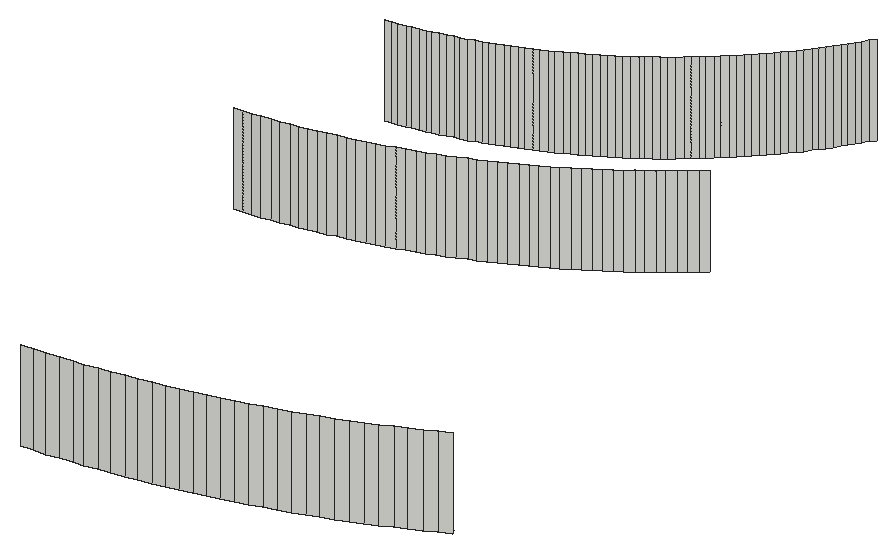
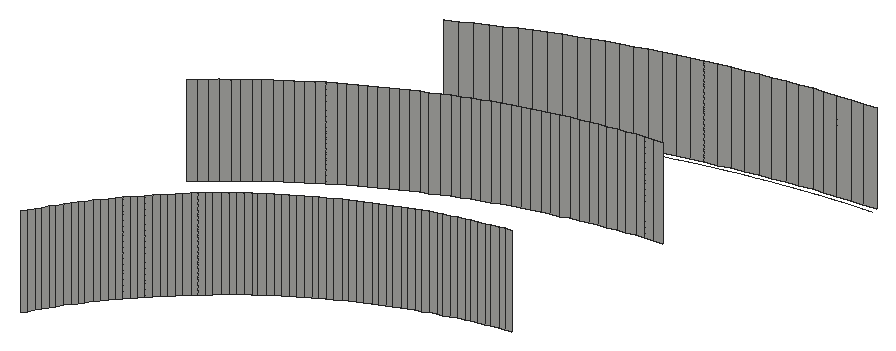
# SketchUp Ruby script. Lengths in inches.
U = 1.inch
M = Sketchup.active_model
def pt(a) = Geom::Point3d.new(a.map { |v| v * U })
def face(e, loops, mat)
  f = e.add_face(loops[0].map { |a| pt(a) })
  loops[1..].each { |l| e.add_face(l.map { |a| pt(a) }).erase! }
  f.material = f.back_material = mat if mat
  f
end
# faces: each face lists its corners as indices into pts; further lists are holes
def faces(e, pts, list, mat = nil) = list.each { |f| face(e, (f[0].is_a?(Array) ? f : [f]).map { |l| l.map { |i| pts[i] } }, mat) }
# xy, xz, yz: faces in a plane at the given z, y or x. An outline is a flat list of corners, or four numbers for a rectangle; further outlines are holes
def ring(l) = l.size == 4 ? [[l[0], l[1]], [l[2], l[1]], [l[2], l[3]], [l[0], l[3]]] : l.each_slice(2).to_a
def flat(e, list, mat, &to3) = list.each { |f| face(e, (f[0].is_a?(Array) ? f : [f]).map { |l| ring(l).map { |u, v| to3.(u, v) } }, mat) }
def xy(e, z, list, mat = nil) = flat(e, list, mat) { |x, y| [x, y, z] }
def xz(e, y, list, mat = nil) = flat(e, list, mat) { |x, z| [x, y, z] }
def yz(e, x, list, mat = nil) = flat(e, list, mat) { |y, z| [x, y, z] }
def lines(e, pts, list) = list.each { |a, b| e.add_line(pt(pts[a]), pt(pts[b])) }
# prism: a flat outline (further loops are holes) pulled along v
def prism(e, loops, v, mat = nil)
  f = face(e, loops, mat); d = Geom::Vector3d.new(v.map { |x| x * U })
  f.pushpull(f.normal.samedirection?(d) ? d.length : -d.length)
end
def box(e, o, s, mat = nil) = prism(e, [[o, [o[0] + s[0], o[1], o[2]], [o[0] + s[0], o[1] + s[1], o[2]], [o[0], o[1] + s[1], o[2]]]], [0, 0, s[2]], mat)
def at(x, y, z, deg = 0) = Geom::Transformation.translation(pt([x, y, z])) * Geom::Transformation.rotation(ORIGIN, Z_AXIS, deg.degrees)
def axes(o, x, y, z) = Geom::Transformation.new([*x, 0, *y, 0, *z, 0, *pt(o).to_a, 1])
def part(name) = M.definitions.add(name)
# library, detail: a bought-in or finely detailed component or shape, given as its bounding box
def library(name, o, s) = part(name).tap { |d| box(d.entities, o, s) }
def detail(e, o, s) = box(e.add_group.entities, o, s)
def put(e, d, t, mat = nil) = e.add_instance(d, t).tap { |i| i.material = mat if mat }
def group(e, t, mat = nil) = e.add_group.tap { |g| g.transformation = t; g.material = mat if mat }.entities
root = M.entities
p = [[177.92,229.04,246],[177.78,229.03,246],[177.78,229.03,247],[177.92,229.04,247],[178.05,229.05,246],[178.05,229.05,247],
  [178.18,229.07,246],[178.18,229.07,247],[178.31,229.09,246],[178.31,229.09,247],[178.43,229.1,246],[178.43,229.1,247],
  [178.5625,229.125,246],[178.5625,229.125,247],[178.69,229.14,246],[178.69,229.14,247],[178.82,229.17,246],[178.82,229.17,247],
  [178.95,229.19,246],[178.95,229.19,247],[179.08,229.22,246],[179.08,229.22,247],[179.21,229.25,246],[179.21,229.25,247],
  [179.33,229.28,246],[179.33,229.28,247],[179.46,229.31,246],[179.46,229.31,247],[179.59,229.34,246],[179.59,229.34,247],
  [179.71,229.375,246],[179.71,229.375,247],[179.84,229.41,246],[179.84,229.41,247],[179.97,229.45,246],[179.97,229.45,247],
  [180.09,229.49,246],[180.09,229.49,247],[180.21,229.53,246],[180.21,229.53,247],[180.34,229.57,246],[180.34,229.57,247],
  [180.46,229.62,246],[180.46,229.62,247],[180.58,229.66,246],[180.58,229.66,247],[180.71,229.71,246],[180.71,229.71,247],
  [180.83,229.76,246],[180.83,229.76,247],[180.95,229.8125,246],[180.95,229.8125,247],[181.07,229.86,246],[181.07,229.86,247],
  [181.1875,229.92,246],[181.1875,229.92,247],[181.31,229.97,246],[181.31,229.97,247],[181.42,230.03,246],[181.42,230.03,247],
  [181.54,230.09,246],[181.54,230.09,247],[181.66,230.15,246],[181.66,230.15,247],[177.82,232.05,248],[177.82,232.05,247],
  [177.73,232.04,247],[177.73,232.04,248],[177.91,232.06,248],[177.91,232.06,247],[178,232.07,248],[178,232.07,247],
  [178.1,232.09,248],[178.1,232.09,247],[178.19,232.1,248],[178.19,232.1,247],[178.28,232.12,248],[178.28,232.12,247],
  [178.37,232.13,248],[178.37,232.13,247],[178.46,232.15,248],[178.46,232.15,247],[178.54,232.17,248],[178.54,232.17,247],
  [178.63,232.19,248],[178.63,232.19,247],[178.72,232.22,248],[178.72,232.22,247],[178.8125,232.24,248],[178.8125,232.24,247],
  [178.9,232.26,248],[178.9,232.26,247],[178.99,232.29,248],[178.99,232.29,247],[179.08,232.31,248],[179.08,232.31,247],
  [179.16,232.34,248],[179.16,232.34,247],[179.25,232.37,248],[179.25,232.37,247],[179.34,232.4,248],[179.34,232.4,247],
  [179.42,232.43,248],[179.42,232.43,247],[179.51,232.46,248],[179.51,232.46,247],[179.59,232.5,248],[179.59,232.5,247],
  [179.68,232.53,248],[179.68,232.53,247],[179.76,232.57,248],[179.76,232.57,247],[179.85,232.61,248],[179.85,232.61,247],
  [179.93,232.64,248],[179.93,232.64,247],[180.01,232.68,248],[180.01,232.68,247],[180.1,232.72,248],[180.1,232.72,247],
  [180.18,232.76,248],[180.18,232.76,247],[180.26,232.81,248],[180.26,232.81,247],[180.34,232.85,248],[180.34,232.85,247],
  [180.42,232.89,248],[180.42,232.89,247],[180.5,232.9375,248],[180.5,232.9375,247],[180.58,232.98,248],[180.58,232.98,247],
  [180.66,233.03,248],[180.66,233.03,247],[180.74,233.08,248],[180.74,233.08,247],[180.8125,233.13,248],[180.8125,233.13,247],
  [180.89,233.18,248],[180.89,233.18,247],[180.96,233.23,248],[180.96,233.23,247],[181.04,233.28,248],[181.04,233.28,247],
  [181.11,233.34,248],[181.11,233.34,247],[181.1875,233.39,248],[181.1875,233.39,247],[181.26,233.45,248],[181.26,233.45,247],
  [181.33,233.5,248],[181.33,233.5,247],[181.41,233.56,248],[181.41,233.56,247],[181.48,233.62,248],[181.48,233.62,247],
  [181.55,233.68,248],[181.55,233.68,247],[181.62,233.74,248],[181.62,233.74,247],[177.78,234.0625,247],[177.85,234.07,247],
  [177.85,234.07,248],[177.78,234.0625,248],[177.91,234.08,247],[177.91,234.08,248],[177.98,234.1,247],[177.98,234.1,248],
  [178.04,234.11,247],[178.04,234.11,248],[178.1,234.125,247],[178.1,234.125,248],[178.17,234.14,247],[178.17,234.14,248],
  [178.23,234.15,247],[178.23,234.15,248],[178.29,234.17,247],[178.29,234.17,248],[178.36,234.1875,247],[178.36,234.1875,248],
  [178.42,234.21,247],[178.42,234.21,248],[178.48,234.22,247],[178.48,234.22,248],[178.55,234.24,247],[178.55,234.24,248],
  [178.61,234.27,247],[178.61,234.27,248],[178.67,234.29,247],[178.67,234.29,248],[178.73,234.31,247],[178.73,234.31,248],
  [178.79,234.33,247],[178.79,234.33,248],[178.85,234.36,247],[178.85,234.36,248],[178.91,234.38,247],[178.91,234.38,248],
  [178.97,234.41,247],[178.97,234.41,248],[179.03,234.43,247],[179.03,234.43,248],[179.09,234.46,247],[179.09,234.46,248],
  [179.15,234.49,247],[179.15,234.49,248],[179.21,234.52,247],[179.21,234.52,248],[179.27,234.54,247],[179.27,234.54,248],
  [179.33,234.58,247],[179.33,234.58,248],[179.39,234.61,247],[179.39,234.61,248],[179.44,234.64,247],[179.44,234.64,248],
  [179.5,234.67,247],[179.5,234.67,248],[179.56,234.7,247],[179.56,234.7,248],[179.61,234.74,247],[179.61,234.74,248],
  [179.67,234.77,247],[179.67,234.77,248],[179.72,234.81,247],[179.72,234.81,248],[179.78,234.84,247],[179.78,234.84,248],
  [179.83,234.88,247],[179.83,234.88,248],[179.89,234.92,247],[179.89,234.92,248],[179.9375,234.95,247],[179.9375,234.95,248],
  [179.99,234.99,247],[179.99,234.99,248],[180.04,235.03,247],[180.04,235.03,248],[180.1,235.07,247],[180.1,235.07,248],
  [180.15,235.11,247],[180.15,235.11,248],[180.2,235.16,247],[180.2,235.16,248],[180.25,235.2,247],[180.25,235.2,248],
  [180.3,235.24,247],[180.3,235.24,248],[180.35,235.28,247],[180.35,235.28,248],[180.39,235.33,247],[180.39,235.33,248],
  [180.44,235.375,247],[180.44,235.375,248],[180.49,235.42,247],[180.49,235.42,248],[180.54,235.46,247],[180.54,235.46,248],
  [180.58,235.51,247],[180.58,235.51,248],[180.625,235.56,247],[180.625,235.56,248],[180.67,235.61,247],[180.67,235.61,248],
  [180.72,235.65,247],[180.72,235.65,248],[180.76,235.7,247],[180.76,235.7,248],[180.8,235.75,247],[180.8,235.75,248],
  [180.84,235.8,247],[180.84,235.8,248],[180.89,235.85,247],[180.89,235.85,248],[180.93,235.9,247],[180.93,235.9,248],
  [180.97,235.96,247],[180.97,235.96,248],[181.01,236.01,247],[181.01,236.01,248],[181.05,236.0625,247],[181.05,236.0625,248],
  [181.08,236.11,247],[181.08,236.11,248],[181.12,236.17,247],[181.12,236.17,248],[181.16,236.22,247],[181.16,236.22,248],
  [181.19,236.28,247],[181.19,236.28,248],[181.23,236.33,247],[181.23,236.33,248],[181.26,236.39,247],[181.26,236.39,248],
  [181.3,236.44,247],[181.3,236.44,248],[181.63,230.2,246],[181.52,230.14,246],[181.4,230.08,246],[181.28,230.02,246],
  [181.16,229.97,246],[181.05,229.91,246],[180.93,229.86,246],[180.81,229.8125,246],[180.69,229.76,246],[180.5625,229.72,246],
  [180.44,229.67,246],[180.32,229.625,246],[180.2,229.58,246],[180.07,229.54,246],[179.95,229.5,246],[179.82,229.46,246],
  [179.7,229.43,246],[179.57,229.39,246],[179.45,229.36,246],[179.32,229.33,246],[179.19,229.3,246],[179.07,229.27,246],
  [178.94,229.25,246],[178.8125,229.22,246],[178.68,229.2,246],[178.56,229.18,246],[178.43,229.16,246],[178.3,229.14,246],
  [178.17,229.125,246],[178.04,229.11,246],[177.91,229.1,246],[177.78,229.09,246]]
faces(root,p,[[0,1,2,3],[4,0,3,5],[6,4,5,7],[8,6,7,9],[10,8,9,11],[12,10,11,13],[14,12,13,15],[16,14,15,17],
  [18,16,17,19],[20,18,19,21],[22,20,21,23],[24,22,23,25],[26,24,25,27],[28,26,27,29],[30,28,29,31],[32,30,31,33],
  [34,32,33,35],[36,34,35,37],[38,36,37,39],[40,38,39,41],[42,40,41,43],[44,42,43,45],[46,44,45,47],[48,46,47,49],
  [50,48,49,51],[52,50,51,53],[54,52,53,55],[56,54,55,57],[58,56,57,59],[60,58,59,61],[62,60,61,63],[64,65,66,67],
  [68,69,65,64],[70,71,69,68],[72,73,71,70],[74,75,73,72],[76,77,75,74],[78,79,77,76],[80,81,79,78],[82,83,81,80],
  [84,85,83,82],[86,87,85,84],[88,89,87,86],[90,91,89,88],[92,93,91,90],[94,95,93,92],[96,97,95,94],[98,99,97,96],
  [100,101,99,98],[102,103,101,100],[104,105,103,102],[106,107,105,104],[108,109,107,106],[110,111,109,108],[112,113,111,110],[114,115,113,112],
  [116,117,115,114],[118,119,117,116],[120,121,119,118],[122,123,121,120],[124,125,123,122],[126,127,125,124],[128,129,127,126],[130,131,129,128],
  [132,133,131,130],[134,135,133,132],[136,137,135,134],[138,139,137,136],[140,141,139,138],[142,143,141,140],[144,145,143,142],[146,147,145,144],
  [148,149,147,146],[150,151,149,148],[152,153,151,150],[154,155,153,152],[156,157,155,154],[158,159,157,156],[160,161,162,163],[161,164,165,162],
  [164,166,167,165],[166,168,169,167],[168,170,171,169],[170,172,173,171],[172,174,175,173],[174,176,177,175],[176,178,179,177],[178,180,181,179],
  [180,182,183,181],[182,184,185,183],[184,186,187,185],[186,188,189,187],[188,190,191,189],[190,192,193,191],[192,194,195,193],[194,196,197,195],
  [196,198,199,197],[198,200,201,199],[200,202,203,201],[202,204,205,203],[204,206,207,205],[206,208,209,207],[208,210,211,209],[210,212,213,211],
  [212,214,215,213],[214,216,217,215],[216,218,219,217],[218,220,221,219],[220,222,223,221],[222,224,225,223],[224,226,227,225],[226,228,229,227],
  [228,230,231,229],[230,232,233,231],[232,234,235,233],[234,236,237,235],[236,238,239,237],[238,240,241,239],[240,242,243,241],[242,244,245,243],
  [244,246,247,245],[246,248,249,247],[248,250,251,249],[250,252,253,251],[252,254,255,253],[254,256,257,255],[256,258,259,257],[258,260,261,259],
  [260,262,263,261],[262,264,265,263],[264,266,267,265],[266,268,269,267],[268,270,271,269],[270,272,273,271],[272,274,275,273],[274,276,277,275],
  [276,278,279,277],[278,280,281,279],[280,282,283,281],[282,284,285,283],[284,286,287,285],[286,288,289,287],[288,290,291,289],[290,292,293,291],
  [292,294,295,293]])
lines(root,p,[[296,297],[297,298],[298,299],[299,300],[300,301],[301,302],[302,303],[303,304],[304,305],[305,306],[306,307],[307,308],
  [308,309],[309,310],[310,311],[311,312],[312,313],[313,314],[314,315],[315,316],[316,317],[317,318],[318,319],[319,320],
  [320,321],[321,322],[322,323],[323,324],[324,325],[325,326],[326,327]])
